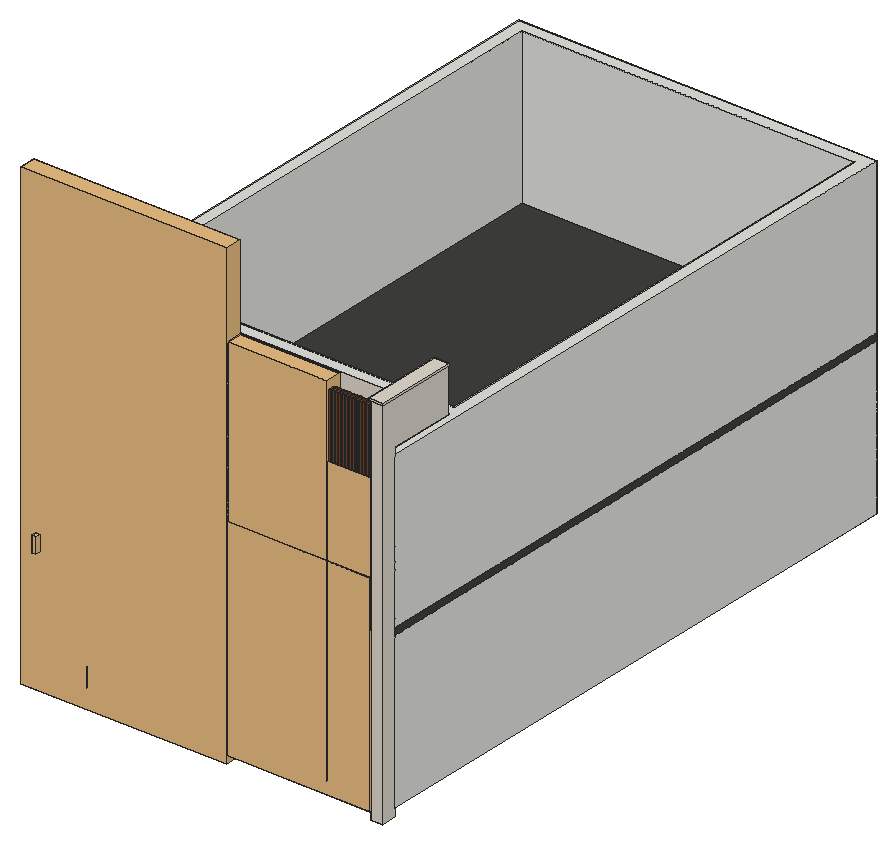
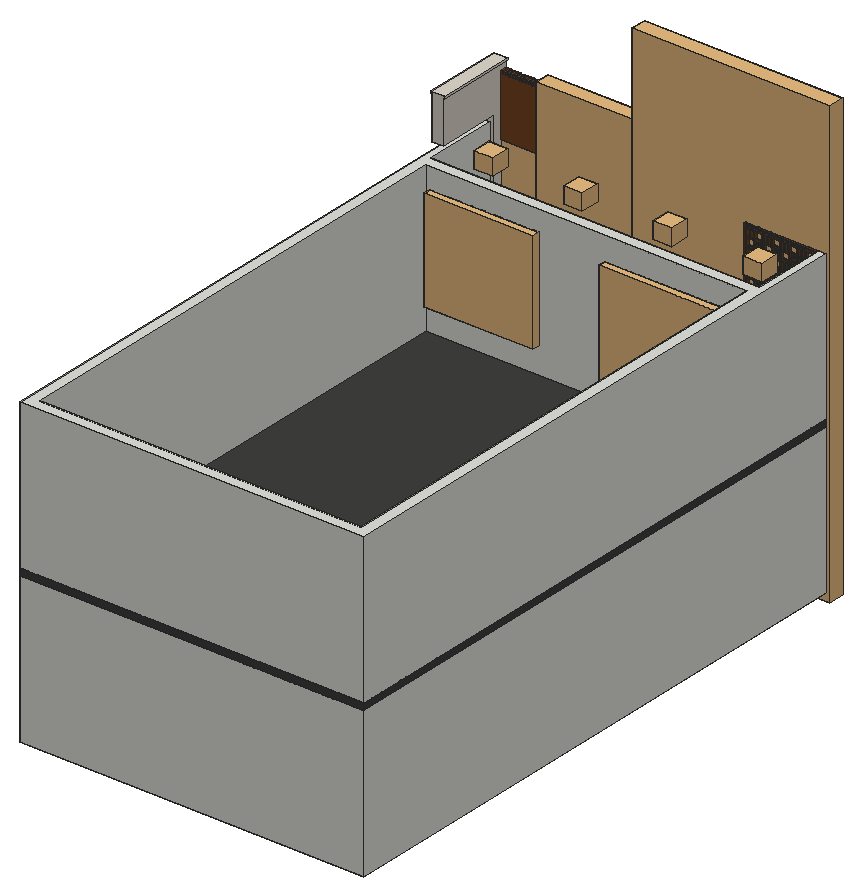
# SketchUp Ruby script. Lengths in inches.
U = 1.inch
M = Sketchup.active_model
def pt(a) = Geom::Point3d.new(a.map { |v| v * U })
def face(e, loops, mat)
  f = e.add_face(loops[0].map { |a| pt(a) })
  loops[1..].each { |l| e.add_face(l.map { |a| pt(a) }).erase! }
  f.material = f.back_material = mat if mat
  f
end
# faces: each face lists its corners as indices into pts; further lists are holes
def faces(e, pts, list, mat = nil) = list.each { |f| face(e, (f[0].is_a?(Array) ? f : [f]).map { |l| l.map { |i| pts[i] } }, mat) }
# xy, xz, yz: faces in a plane at the given z, y or x. An outline is a flat list of corners, or four numbers for a rectangle; further outlines are holes
def ring(l) = l.size == 4 ? [[l[0], l[1]], [l[2], l[1]], [l[2], l[3]], [l[0], l[3]]] : l.each_slice(2).to_a
def flat(e, list, mat, &to3) = list.each { |f| face(e, (f[0].is_a?(Array) ? f : [f]).map { |l| ring(l).map { |u, v| to3.(u, v) } }, mat) }
def xy(e, z, list, mat = nil) = flat(e, list, mat) { |x, y| [x, y, z] }
def xz(e, y, list, mat = nil) = flat(e, list, mat) { |x, z| [x, y, z] }
def yz(e, x, list, mat = nil) = flat(e, list, mat) { |y, z| [x, y, z] }
def lines(e, pts, list) = list.each { |a, b| e.add_line(pt(pts[a]), pt(pts[b])) }
# prism: a flat outline (further loops are holes) pulled along v
def prism(e, loops, v, mat = nil)
  f = face(e, loops, mat); d = Geom::Vector3d.new(v.map { |x| x * U })
  f.pushpull(f.normal.samedirection?(d) ? d.length : -d.length)
end
def box(e, o, s, mat = nil) = prism(e, [[o, [o[0] + s[0], o[1], o[2]], [o[0] + s[0], o[1] + s[1], o[2]], [o[0], o[1] + s[1], o[2]]]], [0, 0, s[2]], mat)
def at(x, y, z, deg = 0) = Geom::Transformation.translation(pt([x, y, z])) * Geom::Transformation.rotation(ORIGIN, Z_AXIS, deg.degrees)
def axes(o, x, y, z) = Geom::Transformation.new([*x, 0, *y, 0, *z, 0, *pt(o).to_a, 1])
def part(name) = M.definitions.add(name)
# library, detail: a bought-in or finely detailed component or shape, given as its bounding box
def library(name, o, s) = part(name).tap { |d| box(d.entities, o, s) }
def detail(e, o, s) = box(e.add_group.entities, o, s)
def put(e, d, t, mat = nil) = e.add_instance(d, t).tap { |i| i.material = mat if mat }
def group(e, t, mat = nil) = e.add_group.tap { |g| g.transformation = t; g.material = mat if mat }.entities
root = M.entities
M.materials.add("1448 AP 8253 RAVEN SONG").color = [64, 64, 63]
M.materials.add("[0135_DarkGray]").color = [81, 81, 81]
M.materials.add("[Concrete Stamped Ashlar]").color = [106, 67, 30]
M.materials.add("[Metal Seamed]").color = [61, 62, 60]
M.materials.add("[Steel Brushed Stainless]").color = [51, 51, 51]
M.materials.add("[Stone Vein Gray]").color = [63, 63, 63]
M.materials.add("[Tile Various Tan]").color = [223, 216, 204]
M.materials.add("[Translucent Glass Blue]1").color = [168, 168, 168]
M.materials["[Translucent Glass Blue]1"].alpha = 0.5
M.materials.add("[Translucent Glass Gray]").color = [181, 181, 181]
M.materials["[Translucent Glass Gray]"].alpha = 0.5
M.materials.add("[Translucent Glass Gray]1").color = [128, 128, 128]
M.materials["[Translucent Glass Gray]1"].alpha = 0.15
M.materials.add("[Wood Veneer 01]").color = [91, 58, 35]
M.materials.add("[Wood Veneer 01]1").color = [120, 70, 37]
c1 = library("Jaali+Partition",[0,0,0],[29.75,4.875,91.45])
c2 = library("Group\#15",[-15,-12.5,0],[147,12.5,163])
c3 = library("Group\#17",[0,0,0],[75,12,279])
c4 = library("Group\#18",[0,-3.5,0],[74,3.5,102])
c5 = library("Group\#20",[-2.91,0,-6],[155.91,13,360])
c6 = part("1")
prism(c6.entities,[[[2,-1,0],[2,1,0],[2,1,48],[2,4,48],[2,4,50],[2,-1,50]]],[-2,0,0])
c7 = library("Group\#72",[0,-2,0],[89,2,34])
c8 = part("Group\#80")
box(c8.entities,[0,-0.5,0],[24,0.5,32.25])
c9 = library("Group\#22",[0,-12.5,0],[72,12.5,15.01])
c10 = library("Curtains",[0,0,0],[121.73,8.19,117.22])
c11 = part("หน้าต่าง3บาน")
xy(c11.entities,42.78,[[77.6875,12.74,148.55,16.68]])
xy(c11.entities,43.96,[[78.87,12.74,147.37,12.74,147.37,14.71,125.72,14.71,125.72,13.13,100.52,13.13,100.52,14.71,78.87,14.71],[100.52,13.13,102.88,14.71],[123.36,13.13,125.72,14.71],[102.49,14.71,123.75,14.71,123.75,16.28,147.37,16.28,147.37,16.68,78.87,16.68,78.87,16.28,102.49,16.28]])
xy(c11.entities,45.93,[[102.49,13.13,123.75,13.92],[102.49,13.92,123.75,14.71],[80.84,14.71,100.52,15.49],[125.72,14.71,145.4,15.49],[80.84,15.49,100.52,16.28],
  [125.72,15.49,145.4,16.28]])
xy(c11.entities,83.09,[[102.49,13.13,123.75,13.92],[102.49,13.92,123.75,14.71],[80.84,14.71,100.52,15.49],[125.72,14.71,145.4,15.49],[80.84,15.49,100.52,16.28],
  [125.72,15.49,145.4,16.28]])
xy(c11.entities,84.91,[[78.87,12.74,78.87,14.71,100.52,14.71,100.52,13.13,125.72,13.13,125.72,14.71,147.37,14.71,147.37,12.74],[100.52,13.13,125.72,14.71],[102.49,14.71,102.49,16.28,78.87,16.28,78.87,16.68,147.37,16.68,147.37,16.28,123.75,16.28,123.75,14.71],[78.87,14.71,102.49,16.28]])
xy(c11.entities,86.09,[[77.6875,12.74,148.55,16.68]])
xz(c11.entities,12.74,[[[77.6875,42.78,148.55,86.09],[78.87,43.96,147.37,84.91]]])
xz(c11.entities,13.13,[[[100.52,43.96,125.72,84.91],[102.49,45.93,123.75,83.09]]])
xz(c11.entities,13.92,[[102.49,45.93,123.75,83.09]],"[Translucent Glass Blue]1")
xz(c11.entities,14.71,[[78.87,43.96,100.52,43.96,100.52,45.93,80.84,45.93,80.84,83.09,100.52,83.09,100.52,84.91,78.87,84.91],[100.52,43.96,102.49,84.91],[102.49,43.96,123.75,45.93],[125.72,43.96,147.37,43.96,147.37,84.91,125.72,84.91,125.72,83.09,145.4,83.09,145.4,45.93,125.72,45.93],[102.49,83.09,123.75,84.91]])
xz(c11.entities,15.49,[[80.44,82.9375,80.84,83.73]])
xz(c11.entities,15.49,[[80.84,45.93,100.52,83.09],[125.72,45.93,145.4,83.09]],"[Translucent Glass Blue]1")
xz(c11.entities,16.28,[[[78.87,43.96,102.49,84.91],[80.84,45.93,100.52,83.09]],[[123.75,43.96,147.37,84.91],[125.72,45.93,145.4,83.09]]])
xz(c11.entities,16.68,[[[77.6875,42.78,148.55,86.09],[78.87,43.96,147.37,84.91]]])
yz(c11.entities,77.6875,[[12.74,42.78,16.68,86.09]])
yz(c11.entities,78.87,[[12.74,43.96,14.71,84.91],[16.28,43.96,16.68,84.91]])
yz(c11.entities,80.84,[[14.71,45.93,15.49,83.09],[15.49,45.93,16.28,83.09]])
yz(c11.entities,100.52,[[13.13,43.96,14.71,84.91],[14.71,45.93,15.49,83.09],[15.49,45.93,16.28,83.09]])
yz(c11.entities,102.49,[[14.71,43.96,16.28,84.91],[13.13,45.93,13.92,83.09],[13.92,45.93,14.71,83.09]])
yz(c11.entities,123.75,[[14.71,43.96,16.28,84.91],[13.13,45.93,13.92,83.09],[13.92,45.93,14.71,83.09]])
yz(c11.entities,125.72,[[13.13,43.96,14.71,84.91],[14.71,45.93,15.49,83.09],[15.49,45.93,16.28,83.09]])
yz(c11.entities,145.4,[[14.71,45.93,15.49,83.09],[15.49,45.93,16.28,83.09]])
yz(c11.entities,147.37,[[12.74,43.96,14.71,84.91],[16.28,43.96,16.68,84.91]])
yz(c11.entities,148.55,[[12.74,42.78,16.68,86.09]])
p = [[80.44,15.49,84.91],[80.44,15.49,83.73]]
lines(c11.entities,p,[[0,1]])
c12 = library("AS-120-mm\#1",[0,0,0],[49.44,4.72,60])
c13 = library("WALL LIGHT 69",[4.19,4.05,-8.78],[4.61,5.7,17.13])
c14 = part("Group\#81")
prism(c14.entities,[[[8,8,0],[8,0,0],[0,0,0],[0,8,0]],[[4.25,3.75,0],[4.25,0.5,0],[7.5,0.5,0],[7.5,3.75,0]],[[0.5,7.5,0],[0.5,4.25,0],[3.75,4.25,0],[3.75,7.5,0]],[[5.625,4.25,0],[5.625,7.5,0],[4.25,7.5,0],[4.25,4.25,0]],[[7.5,7.5,0],[6.125,7.5,0],[6.125,4.25,0],[7.5,4.25,0]],[[0.5,3.75,0],[0.5,2.375,0],[3.75,2.375,0],[3.75,3.75,0]],[[0.5,0.5,0],[3.75,0.5,0],[3.75,1.875,0],[0.5,1.875,0]]],[0,0,3])
c15 = part("contemporary square jaali - swamy and co")
g1 = group(c15.entities,at(69.36,8.01,-1.33))
put(g1,c14,axes([24,1.28,40],[1,0,0],[0,0,1],[0,-0.42667,0]),"[Concrete Stamped Ashlar]")
put(g1,c14,axes([0,1.28,48],[1,0,0],[0,0,1],[0,-0.42667,0]),"[Concrete Stamped Ashlar]")
put(g1,c14,axes([8,1.28,40],[1,0,0],[0,0,1],[0,-0.42667,0]),"[Concrete Stamped Ashlar]")
put(g1,c14,axes([16,1.28,40],[1,0,0],[0,0,1],[0,-0.42667,0]),"[Concrete Stamped Ashlar]")
put(g1,c14,axes([8,1.28,48],[1,0,0],[0,0,1],[0,-0.42667,0]),"[Concrete Stamped Ashlar]")
put(g1,c14,axes([24,1.28,48],[1,0,0],[0,0,1],[0,-0.42667,0]),"[Concrete Stamped Ashlar]")
put(g1,c14,axes([16,1.28,48],[1,0,0],[0,0,1],[0,-0.42667,0]),"[Concrete Stamped Ashlar]")
put(g1,c14,axes([0,1.28,32],[1,0,0],[0,0,1],[0,-0.42667,0]),"[Concrete Stamped Ashlar]")
put(g1,c14,axes([8,1.28,24],[1,0,0],[0,0,1],[0,-0.42667,0]),"[Concrete Stamped Ashlar]")
put(g1,c14,axes([16,1.28,24],[1,0,0],[0,0,1],[0,-0.42667,0]),"[Concrete Stamped Ashlar]")
put(g1,c14,axes([24,1.28,24],[1,0,0],[0,0,1],[0,-0.42667,0]),"[Concrete Stamped Ashlar]")
put(g1,c14,axes([24,1.28,56],[1,0,0],[0,0,1],[0,-0.42667,0]),"[Concrete Stamped Ashlar]")
put(g1,c14,axes([16,1.28,8],[1,0,0],[0,0,1],[0,-0.42667,0]),"[Concrete Stamped Ashlar]")
put(g1,c14,axes([0,1.28,24],[1,0,0],[0,0,1],[0,-0.42667,0]),"[Concrete Stamped Ashlar]")
put(g1,c14,axes([0,1.28,16],[1,0,0],[0,0,1],[0,-0.42667,0]),"[Concrete Stamped Ashlar]")
put(g1,c14,axes([24,1.28,8],[1,0,0],[0,0,1],[0,-0.42667,0]),"[Concrete Stamped Ashlar]")
put(g1,c14,axes([8,1.28,16],[1,0,0],[0,0,1],[0,-0.42667,0]),"[Concrete Stamped Ashlar]")
put(g1,c14,axes([16,1.28,16],[1,0,0],[0,0,1],[0,-0.42667,0]),"[Concrete Stamped Ashlar]")
put(g1,c14,axes([24,1.28,16],[1,0,0],[0,0,1],[0,-0.42667,0]),"[Concrete Stamped Ashlar]")
put(g1,c14,axes([0,1.28,56],[1,0,0],[0,0,1],[0,-0.42667,0]),"[Concrete Stamped Ashlar]")
put(g1,c14,axes([24,1.28,32],[1,0,0],[0,0,1],[0,-0.42667,0]),"[Concrete Stamped Ashlar]")
put(g1,c14,axes([16,1.28,32],[1,0,0],[0,0,1],[0,-0.42667,0]),"[Concrete Stamped Ashlar]")
put(g1,c14,axes([0,1.28,40],[1,0,0],[0,0,1],[0,-0.42667,0]),"[Concrete Stamped Ashlar]")
put(g1,c14,axes([8,1.28,32],[1,0,0],[0,0,1],[0,-0.42667,0]),"[Concrete Stamped Ashlar]")
put(g1,c14,axes([0,1.28,0],[1,0,0],[0,0,1],[0,-0.42667,0]),"[Concrete Stamped Ashlar]")
put(g1,c14,axes([0,1.28,8],[1,0,0],[0,0,1],[0,-0.42667,0]),"[Concrete Stamped Ashlar]")
put(g1,c14,axes([16,1.28,56],[1,0,0],[0,0,1],[0,-0.42667,0]),"[Concrete Stamped Ashlar]")
put(g1,c14,axes([8,1.28,0],[1,0,0],[0,0,1],[0,-0.42667,0]),"[Concrete Stamped Ashlar]")
put(g1,c14,axes([16,1.28,0],[1,0,0],[0,0,1],[0,-0.42667,0]),"[Concrete Stamped Ashlar]")
put(g1,c14,axes([24,1.28,0],[1,0,0],[0,0,1],[0,-0.42667,0]),"[Concrete Stamped Ashlar]")
put(g1,c14,axes([8,1.28,56],[1,0,0],[0,0,1],[0,-0.42667,0]),"[Concrete Stamped Ashlar]")
put(g1,c14,axes([8,1.28,8],[1,0,0],[0,0,1],[0,-0.42667,0]),"[Concrete Stamped Ashlar]")
g2 = group(c15.entities,at(67.86,7.61,-2.83),"[Wood Veneer 01]")
xy(g2,0.5,[[0.5,0,34.5,2]])
xy(g2,1.5,[[1.5,0,33.5,2]])
xy(g2,65.5,[[1.5,0,33.5,2]])
xy(g2,66.5,[[0.5,0,34.5,2]])
xz(g2,0,[[[0.5,0.5,34.5,66.5],[1.5,1.5,33.5,65.5]]])
yz(g2,0.5,[[0,0.5,2,66.5]])
yz(g2,1.5,[[0,1.5,2,65.5]])
yz(g2,33.5,[[0,1.5,2,65.5]])
yz(g2,34.5,[[0,0.5,2,66.5]])
c16 = part("PENTEK_RP Fineline 50S_Sliding_DoorCase_E1")
box(c16.entities,[0,0,0],[1.51,3.66,99.27],"[0135_DarkGray]")
c17 = part("PENTEK_RP Fineline 50S_SlidingDooe_Case_E2")
box(c17.entities,[0,0,0],[96.25,3.66,1.51],"[0135_DarkGray]")
c18 = part("pentek_RP Fineline 50S_SlidingDoor_Case")
put(c18.entities,c16,at(97.76,0,0))
put(c18.entities,c17,at(1.51,0,0))
put(c18.entities,c16,at(0,0,0))
put(c18.entities,c17,at(1.51,0,97.76))
c19 = part("PENTEK_RP Fineline 50S_SlidingDoor_GlazingBead_2")
box(c19.entities,[0,0,0],[0.56,0.59,94.39],"[0135_DarkGray]")
c20 = part("PENTEK_RP Fineline 50S_SlidingDoor_Glass")
box(c20.entities,[0,0,0],[46.58,0.16,94.39],"[Translucent Glass Gray]1")
c21 = part("PENTEK_RP Fineline 50S_SlidingDoor_GlazingBead")
box(c21.entities,[0,0,0],[45.47,0.59,0.56],"[0135_DarkGray]")
c22 = part("PENTEK_RP Fineline 50S_SlidingDoor_Leaf_E1")
xy(c22.entities,0,[[0,0,0.93,1.97],[0.93,1.57,1.49,1.97]],"[0135_DarkGray]")
xy(c22.entities,96.25,[[0,0,0.93,0,0.93,1.57,1.49,1.57,1.49,1.97,0,1.97]],"[0135_DarkGray]")
xz(c22.entities,0,[[0,0,0.93,96.25]],"[0135_DarkGray]")
xz(c22.entities,1.57,[[0.93,0,1.49,95.32],[0.93,95.32,1.49,96.25]],"[0135_DarkGray]")
xz(c22.entities,1.97,[[0,0,1.49,96.25]],"[0135_DarkGray]")
yz(c22.entities,0,[[0,0,1.97,96.25]],"[0135_DarkGray]")
yz(c22.entities,0.93,[[0,0,1.57,0.93],[0,0.93,1.57,95.32],[0,95.32,1.57,96.25]],"[0135_DarkGray]")
yz(c22.entities,1.49,[[1.57,0,1.97,95.32],[1.57,95.32,1.97,96.25]],"[0135_DarkGray]")
c23 = part("PENTEK_RP Fineline 50S_SlidingDoor_Leaf_E2")
xy(c23.entities,0,[[0,0,0,1.57,0.56,1.57,0.56,1.97,46.02,1.97,46.02,1.57,46.58,1.57,46.58,0]],"[0135_DarkGray]")
xy(c23.entities,0.93,[[0,0,46.58,1.57]],"[0135_DarkGray]")
xy(c23.entities,1.49,[[0.56,1.57,46.02,1.97]],"[0135_DarkGray]")
xz(c23.entities,0,[[0,0,46.58,0.93]],"[0135_DarkGray]")
xz(c23.entities,1.57,[[0,0,0.56,0.93],[46.02,0,46.58,0.93],[0.56,0.93,46.02,1.49]],"[0135_DarkGray]")
xz(c23.entities,1.97,[[0.56,0,46.02,1.49]],"[0135_DarkGray]")
yz(c23.entities,0,[[0,0,1.57,0.93]],"[0135_DarkGray]")
yz(c23.entities,0.56,[[1.57,0,1.97,0.93],[1.57,0.93,1.97,1.49]],"[0135_DarkGray]")
yz(c23.entities,46.02,[[1.57,0,1.97,0.93],[1.57,0.93,1.97,1.49]],"[0135_DarkGray]")
yz(c23.entities,46.58,[[0,0,1.57,0.93]],"[0135_DarkGray]")
c24 = part("PENTEK_RP Fineline S_SlidingDoor_Leaf1")
put(c24.entities,c19,at(0.93,0,0.93))
put(c24.entities,c19,at(46.96,0,0.93))
put(c24.entities,c20,at(1.49,1.42,0.93))
put(c24.entities,c21,at(1.49,0,0.93))
put(c24.entities,c20,at(1.49,0.59,0.93))
put(c24.entities,c22,at(0,0,0))
put(c24.entities,c22,axes([48.44,0,0],[-1,0,0],[0,1,0],[0,0,1]))
put(c24.entities,c23,axes([0.93,0,96.25],[1,0,0],[0,1,0],[0,0,-1]))
put(c24.entities,c23,at(0.93,0,0))
put(c24.entities,c21,at(1.49,0,94.77))
c25 = part("PENTEK_RP Fineline 50S_SlidingDoor_Leaf2")
put(c25.entities,c20,at(1.49,1.42,0.93))
put(c25.entities,c21,at(1.49,0,94.77))
put(c25.entities,c19,at(46.96,0,0.93))
put(c25.entities,c20,at(1.49,0.59,0.93))
put(c25.entities,c19,at(0.93,0,0.93))
put(c25.entities,c22,at(0,0,0))
put(c25.entities,c22,axes([48.44,0,0],[-1,0,0],[0,1,0],[0,0,1]))
put(c25.entities,c21,at(1.49,0,0.93))
put(c25.entities,c23,axes([0.93,0,96.25],[1,0,0],[0,1,0],[0,0,-1]))
put(c25.entities,c23,at(0.93,0,0))
c26 = part("PENTEK_RP+Fineline+50S_Sliding_Door (1)")
put(c26.entities,c18,at(0,-1.88,-0.09))
put(c26.entities,c24,at(1.51,-2.27,1.42))
put(c26.entities,c25,at(49.32,-0.3,1.42))
c27 = library("AS-120-mm",[0,0,0],[49.44,4.72,66.14])
c28 = library("11",[-5.64,-5.64,-13.23],[15.28,15.28,13.23])
xy(root,123,[[39.35,204,39.27,204.01,39.19,204.01,39.12,204.02,38.88,204.05,38.81,204.07,38.65,204.11,38.58,204.13,38.5,204.15,38.36,204.21,38.28,204.24,38.14,204.3,38.07,204.34,37.93,204.41,37.87,204.45,37.8,204.5,37.73,204.54,37.67,204.59,37.61,204.63,37.43,204.78,37.37,204.84,37.3125,204.89,37.26,204.95,37.01,205.25,36.97,205.32,36.92,205.38,36.8,205.59,36.77,205.66,36.73,205.73,36.64,205.94,36.62,206.02,36.59,206.09,36.57,206.17,36.55,206.24,36.51,206.4,36.5,206.47,36.48,206.55,36.46,206.71,36.46,206.79,36.45,206.86,36.45,207.1,36.46,207.18,36.46,207.26,36.47,207.33,36.5,207.57,36.52,207.64,36.56,207.8,36.58,207.87,36.6,207.95,36.66,208.09,36.6875,208.17,36.72,208.24,36.75,208.31,36.79,208.38,36.82,208.45,36.86,208.52,36.9,208.58,36.95,208.65,36.99,208.72,37.04,208.78,37.08,208.84,37.23,209.02,37.29,209.08,37.34,209.14,37.64,209.39,37.7,209.4375,37.77,209.48,37.83,209.53,38.04,209.65,38.11,209.68,38.18,209.72,38.39,209.81,38.47,209.83,38.54,209.86,38.62,209.88,38.69,209.9,38.77,209.92,38.85,209.9375,38.92,209.95,39,209.97,39.16,209.99,39.24,209.99,39.3125,210,39.55,210,39.63,209.99,39.71,209.99,39.78,209.98,40.02,209.95,40.09,209.93,40.25,209.89,40.32,209.87,40.4,209.85,40.54,209.79,40.62,209.76,40.6875,209.73,40.76,209.7,40.83,209.66,40.97,209.59,41.03,209.55,41.1,209.5,41.17,209.46,41.23,209.41,41.29,209.37,41.47,209.22,41.53,209.16,41.59,209.11,41.89,208.75,41.93,208.68,41.98,208.62,42.1,208.41,42.13,208.34,42.17,208.27,42.26,208.06,42.28,207.98,42.31,207.91,42.33,207.83,42.35,207.76,42.39,207.6,42.4,207.53,42.42,207.45,42.43,207.37,42.4375,207.29,42.44,207.21,42.45,207.14,42.45,206.9,42.44,206.82,42.4375,206.74,42.43,206.67,42.4,206.43,42.38,206.36,42.34,206.2,42.32,206.13,42.3,206.05,42.24,205.91,42.21,205.83,42.15,205.69,42.11,205.62,42.08,205.55,42.04,205.48,42,205.42,41.95,205.35,41.91,205.28,41.86,205.22,41.82,205.16,41.67,204.98,41.61,204.92,41.56,204.86,41.26,204.61,41.2,204.5625,41.13,204.52,41.07,204.47,40.86,204.35,40.79,204.32,40.72,204.28,40.51,204.19,40.43,204.17,40.36,204.14,40.28,204.12,40.21,204.1,40.13,204.08,40.05,204.0625,39.98,204.05,39.9,204.03,39.74,204.01,39.66,204.01,39.59,204],[77.87,204,77.79,204.01,77.71,204.01,77.64,204.02,77.4,204.05,77.33,204.07,77.17,204.11,77.1,204.13,77.02,204.15,76.95,204.18,76.8,204.24,76.66,204.3,76.59,204.34,76.45,204.41,76.39,204.45,76.32,204.5,76.25,204.54,76.19,204.59,76.13,204.63,75.95,204.78,75.89,204.84,75.83,204.89,75.68,205.07,75.625,205.13,75.58,205.19,75.53,205.25,75.49,205.32,75.44,205.38,75.32,205.59,75.29,205.66,75.25,205.73,75.16,205.94,75.14,206.02,75.11,206.09,75.09,206.17,75.07,206.24,75.03,206.4,75.02,206.47,75,206.55,74.98,206.71,74.98,206.79,74.97,206.86,74.97,207.1,74.98,207.18,74.98,207.26,74.99,207.33,75.02,207.57,75.04,207.64,75.08,207.8,75.1,207.87,75.125,207.95,75.15,208.02,75.18,208.09,75.21,208.17,75.27,208.31,75.31,208.38,75.34,208.45,75.38,208.52,75.42,208.58,75.47,208.65,75.51,208.72,75.56,208.78,75.6,208.84,75.75,209.02,75.81,209.08,75.86,209.14,76.16,209.39,76.22,209.4375,76.29,209.48,76.35,209.53,76.56,209.65,76.625,209.68,76.7,209.72,76.91,209.81,76.99,209.83,77.0625,209.86,77.14,209.88,77.21,209.9,77.29,209.92,77.37,209.9375,77.44,209.95,77.52,209.97,77.68,209.99,77.76,209.99,77.83,210,78.07,210,78.15,209.99,78.23,209.99,78.3,209.98,78.54,209.95,78.61,209.93,78.77,209.89,78.84,209.87,78.92,209.85,78.99,209.82,79.0625,209.79,79.14,209.76,79.28,209.7,79.35,209.66,79.49,209.59,79.55,209.55,79.62,209.5,79.6875,209.46,79.75,209.41,79.8125,209.37,79.875,209.32,79.93,209.27,79.99,209.22,80.05,209.16,80.11,209.11,80.26,208.93,80.3125,208.87,80.36,208.81,80.41,208.75,80.45,208.68,80.5,208.62,80.62,208.41,80.65,208.34,80.6875,208.27,80.72,208.2,80.78,208.06,80.8,207.98,80.83,207.91,80.85,207.83,80.875,207.76,80.89,207.68,80.91,207.6,80.92,207.53,80.9375,207.45,80.95,207.37,80.96,207.29,80.96,207.21,80.97,207.14,80.97,206.9,80.96,206.82,80.96,206.74,80.95,206.67,80.92,206.43,80.9,206.36,80.86,206.2,80.84,206.13,80.82,206.05,80.76,205.91,80.73,205.83,80.67,205.69,80.63,205.62,80.6,205.55,80.56,205.48,80.52,205.42,80.47,205.35,80.43,205.28,80.38,205.22,80.34,205.16,80.24,205.04,80.1875,204.98,80.13,204.92,80.08,204.86,79.78,204.61,79.72,204.5625,79.65,204.52,79.59,204.47,79.38,204.35,79.3125,204.32,79.24,204.28,79.03,204.19,78.95,204.17,78.88,204.14,78.8,204.12,78.73,204.1,78.65,204.08,78.57,204.0625,78.5,204.05,78.42,204.03,78.26,204.01,78.18,204.01,78.11,204]],"1448 AP 8253 RAVEN SONG")
xy(root,126,[[9.27,183,278.1,183,278.1,195,287.37,195,287.37,663,9.27,663]],"1448 AP 8253 RAVEN SONG")
xz(root,209.99,[[39.16,120,39.24,123],[39.63,120,39.71,123]],"1448 AP 8253 RAVEN SONG")
xz(root,210,[[39.3125,120,39.39,123],[39.39,120,39.47,123],[39.47,120,39.55,123]],"1448 AP 8253 RAVEN SONG")
yz(root,36.45,[[206.86,120,206.94,123],[206.94,120,207.02,123],[207.02,120,207.1,123]],"1448 AP 8253 RAVEN SONG")
yz(root,36.46,[[206.71,120,206.79,123],[207.18,120,207.26,123]],"1448 AP 8253 RAVEN SONG")
p = [[37.06,205.19,120],[37.01,205.25,120],[37.01,205.25,123],[37.06,205.19,123],[36.97,205.32,120],[36.92,205.38,120],
  [36.92,205.38,123],[36.97,205.32,123],[36.88,205.45,120],[36.88,205.45,123],[36.84,205.52,120],[36.84,205.52,123],
  [36.8,205.59,120],[36.8,205.59,123],[36.77,205.66,120],[36.77,205.66,123],[36.73,205.73,120],[36.73,205.73,123],
  [36.7,205.8,120],[36.7,205.8,123],[36.67,205.87,120],[36.67,205.87,123],[36.64,205.94,120],[36.64,205.94,123],
  [36.62,206.02,120],[36.62,206.02,123],[36.59,206.09,120],[36.59,206.09,123],[36.57,206.17,120],[36.57,206.17,123],
  [36.55,206.24,120],[36.55,206.24,123],[36.53,206.32,120],[36.53,206.32,123],[36.51,206.4,120],[36.51,206.4,123],
  [36.5,206.47,120],[36.5,206.47,123],[36.48,206.55,120],[36.48,206.55,123],[36.47,206.63,120],[36.47,206.63,123],
  [36.46,206.71,120],[36.46,206.71,123],[36.46,206.79,120],[36.45,206.86,120],[36.45,206.86,123],[36.46,206.79,123],
  [36.45,207.1,120],[36.46,207.18,120],[36.46,207.18,123],[36.45,207.1,123],[36.46,207.26,120],[36.47,207.33,120],
  [36.47,207.33,123],[36.46,207.26,123],[36.48,207.41,120],[36.48,207.41,123],[36.49,207.49,120],[36.49,207.49,123],
  [36.5,207.57,120],[36.5,207.57,123],[36.52,207.64,120],[36.52,207.64,123],[36.54,207.72,120],[36.54,207.72,123],
  [36.56,207.8,120],[36.56,207.8,123],[36.58,207.87,120],[36.58,207.87,123],[36.6,207.95,120],[36.6,207.95,123],
  [36.63,208.02,120],[36.63,208.02,123],[36.66,208.09,120],[36.66,208.09,123],[36.6875,208.17,120],[36.6875,208.17,123],
  [36.72,208.24,120],[36.72,208.24,123],[36.75,208.31,120],[36.75,208.31,123],[36.79,208.38,120],[36.79,208.38,123],
  [36.82,208.45,120],[36.82,208.45,123],[36.86,208.52,120],[36.86,208.52,123],[36.9,208.58,120],[36.9,208.58,123],
  [36.95,208.65,120],[36.95,208.65,123],[36.99,208.72,120],[36.99,208.72,123],[37.04,208.78,120],[37.04,208.78,123],
  [37.08,208.84,120],[37.08,208.84,123],[37.13,208.9,120],[37.13,208.9,123],[37.18,208.96,120],[37.18,208.96,123],
  [37.23,209.02,120],[37.23,209.02,123],[37.29,209.08,120],[37.29,209.08,123],[37.34,209.14,120],[37.34,209.14,123],
  [37.4,209.19,120],[37.4,209.19,123],[37.46,209.24,120],[37.46,209.24,123],[37.52,209.29,120],[37.52,209.29,123],
  [37.58,209.34,120],[37.58,209.34,123],[37.64,209.39,120],[37.64,209.39,123],[37.7,209.4375,120],[37.7,209.4375,123],
  [37.77,209.48,120],[37.77,209.48,123],[41.17,209.46,120],[41.23,209.41,120],[41.23,209.41,123],[41.17,209.46,123],
  [37.83,209.53,120],[37.83,209.53,123],[37.9,209.57,120],[37.9,209.57,123],[40.97,209.59,120],[41.03,209.55,120],
  [41.03,209.55,123],[40.97,209.59,123],[41.1,209.5,120],[41.1,209.5,123],[37.97,209.61,120],[37.97,209.61,123],
  [38.04,209.65,120],[38.04,209.65,123],[38.11,209.68,120],[38.11,209.68,123],[40.83,209.66,120],[40.9,209.625,120],
  [40.9,209.625,123],[40.83,209.66,123],[38.18,209.72,120],[38.18,209.72,123],[38.25,209.75,120],[38.25,209.75,123],
  [38.32,209.78,120],[38.32,209.78,123],[40.62,209.76,120],[40.6875,209.73,120],[40.6875,209.73,123],[40.62,209.76,123],
  [40.76,209.7,120],[40.76,209.7,123],[38.39,209.81,120],[38.39,209.81,123],[38.47,209.83,120],[38.47,209.83,123],
  [38.54,209.86,120],[38.54,209.86,123],[40.32,209.87,120],[40.4,209.85,120],[40.4,209.85,123],[40.32,209.87,123],
  [40.47,209.82,120],[40.47,209.82,123],[40.54,209.79,120],[40.54,209.79,123],[38.62,209.88,120],[38.62,209.88,123],
  [38.69,209.9,120],[38.69,209.9,123],[38.77,209.92,120],[38.77,209.92,123],[38.85,209.9375,120],[38.85,209.9375,123],
  [38.92,209.95,120],[38.92,209.95,123],[39.94,209.96,120],[40.02,209.95,120],[40.02,209.95,123],[39.94,209.96,123],
  [40.09,209.93,120],[40.09,209.93,123],[40.17,209.91,120],[40.17,209.91,123],[40.25,209.89,120],[40.25,209.89,123],
  [39,209.97,120],[39,209.97,123],[39.08,209.98,120],[39.08,209.98,123],[39.16,209.99,120],[39.16,209.99,123],
  [39.24,209.99,120],[39.3125,210,120],[39.3125,210,123],[39.24,209.99,123],[39.55,210,120],[39.63,209.99,120],
  [39.63,209.99,123],[39.55,210,123],[39.71,209.99,120],[39.78,209.98,120],[39.78,209.98,123],[39.71,209.99,123],
  [39.86,209.97,120],[39.86,209.97,123]]
faces(root,p,[[0,1,2,3],[4,5,6,7],[1,4,7,2],[5,8,9,6],[8,10,11,9],[10,12,13,11],[12,14,15,13],[14,16,17,15],
  [16,18,19,17],[18,20,21,19],[20,22,23,21],[22,24,25,23],[24,26,27,25],[26,28,29,27],[28,30,31,29],[30,32,33,31],
  [32,34,35,33],[34,36,37,35],[36,38,39,37],[38,40,41,39],[40,42,43,41],[44,45,46,47],[48,49,50,51],[52,53,54,55],
  [53,56,57,54],[56,58,59,57],[58,60,61,59],[60,62,63,61],[62,64,65,63],[64,66,67,65],[66,68,69,67],[68,70,71,69],
  [70,72,73,71],[72,74,75,73],[74,76,77,75],[76,78,79,77],[78,80,81,79],[80,82,83,81],[82,84,85,83],[84,86,87,85],
  [86,88,89,87],[88,90,91,89],[90,92,93,91],[92,94,95,93],[94,96,97,95],[96,98,99,97],[98,100,101,99],[100,102,103,101],
  [102,104,105,103],[104,106,107,105],[106,108,109,107],[108,110,111,109],[110,112,113,111],[112,114,115,113],[114,116,117,115],[116,118,119,117],
  [118,120,121,119],[122,123,124,125],[120,126,127,121],[126,128,129,127],[130,131,132,133],[131,134,135,132],[134,122,125,135],[128,136,137,129],
  [136,138,139,137],[138,140,141,139],[142,143,144,145],[143,130,133,144],[140,146,147,141],[146,148,149,147],[148,150,151,149],[152,153,154,155],
  [153,156,157,154],[156,142,145,157],[150,158,159,151],[158,160,161,159],[160,162,163,161],[164,165,166,167],[165,168,169,166],[168,170,171,169],
  [170,152,155,171],[162,172,173,163],[172,174,175,173],[174,176,177,175],[176,178,179,177],[178,180,181,179],[182,183,184,185],[183,186,187,184],
  [186,188,189,187],[188,190,191,189],[190,164,167,191],[180,192,193,181],[192,194,195,193],[194,196,197,195],[198,199,200,201],[202,203,204,205],
  [206,207,208,209],[207,210,211,208],[210,182,185,211]],"1448 AP 8253 RAVEN SONG")
g3 = group(root,at(9.27,183,126))
xy(g3,0,[[[0,12,278.1,480],[9.27,21,268.83,471]]])
xy(g3,30,[[49.44,12,123.6,21],[176.13,12,225.57,21]])
xy(g3,90,[[49.44,12,123.6,21],[176.13,12,225.57,21]])
xy(g3,120,[[[0,12,278.1,480],[9.27,21,268.83,471]]])
xz(g3,12,[[[0,0,278.1,120],[49.44,30,123.6,90],[176.13,30,225.57,90]]],"[Tile Various Tan]")
xz(g3,21,[[[9.27,0,268.83,120],[49.44,30,123.6,90],[176.13,30,225.57,90]]])
xz(g3,471,[[9.27,0,268.83,120]])
xz(g3,480,[[0,0,278.1,120]])
yz(g3,0,[[12,0,480,120]])
yz(g3,9.27,[[21,0,471,120]])
yz(g3,49.44,[[12,30,21,90]])
yz(g3,123.6,[[12,30,21,90]])
yz(g3,176.13,[[12,30,21,90]])
yz(g3,225.57,[[12,30,21,90]])
yz(g3,268.83,[[21,0,471,120]])
yz(g3,278.1,[[12,0,480,120]])
g4 = group(g3,at(0,12,0),"[Tile Various Tan]")
xy(g4,-6,[[268.83,-12,278.1,0]])
xy(g4,252,[[268.83,0,278.1,51]])
xy(g4,286.5,[[267.8,-13,267.8,51,268.83,51,268.83,-12,278.1,-12,278.1,51,279.13,51,279.13,-13]])
xy(g4,288,[[267.8,-13,279.13,51]])
xz(g4,-13,[[267.8,286.5,279.13,288]])
xz(g4,-12,[[268.83,-6,278.1,286.5]],"[Tile Various Tan]")
xz(g4,0,[[268.83,-6,278.1,252]])
xz(g4,51,[[268.83,252,278.1,288],[267.8,286.5,268.83,288],[278.1,286.5,279.13,288]])
yz(g4,267.8,[[-13,286.5,51,288]])
yz(g4,268.83,[[-12,-6,-12,286.5,51,286.5,51,252,0,252,0,-6]],"[Tile Various Tan]")
yz(g4,278.1,[[-12,-6,0,-6,0,252,51,252,51,286.5,-12,286.5]])
yz(g4,279.13,[[-13,286.5,51,288]])
p = [[123.6,0,90],[123.6,0,30],[176.13,0,30],[176.13,0,90],[225.57,0,90],[225.57,0,30]]
lines(g4,p,[[0,1],[2,3],[4,3],[5,4],[2,5]])
put(g4,c1,axes([234.84,-12,126],[1.14262,0,0],[0,1,0],[0,0,1.15906]))
put(g4,c2,axes([132.87,0,0],[1.03,0,0],[0,1,0],[0,0,1]),"[Stone Vein Gray]")
put(g4,c3,axes([157.59,-12,9],[1.03,0,0],[0,1,0],[0,0,1]))
put(g4,c4,axes([176.13,0,9],[1.03,0,0],[0,1,0],[0,0,1]),"[Wood Veneer 01]1")
g5 = group(g4,at(176.13,0,9),"[Tile Various Tan]")
detail(g5,[0,-10.5,0],[92.7,10.5,117])
put(g4,c5,axes([0,-13,0],[1.03,0,0],[0,1,0],[0,0,1]))
g6 = group(g4,at(132.87,-13,0),"[Tile Various Tan]")
box(g6,[-108.15,1,0],[108.15,11,8.99])
g7 = group(g4,at(234.84,-12,232),"[Wood Veneer 01]1")
xy(g7,0,[[0,3,33.99,6]])
xy(g7,48,[[0,3,33.99,6]])
xz(g7,3,[[0,0,33.99,48]])
xz(g7,6,[[0,0,33.99,48]])
yz(g7,0,[[3,0,6,48]])
yz(g7,33.99,[[3,0,6,48]])
put(g7,c6,axes([0,2,0],[1.11023,0,0],[0,1,0],[0,0,1]))
put(g7,c6,axes([2.65,2,0],[1.11023,0,0],[0,1,0],[0,0,1]))
put(g7,c6,axes([5.29,2,0],[1.11023,0,0],[0,1,0],[0,0,1]))
put(g7,c6,axes([7.94,2,0],[1.11023,0,0],[0,1,0],[0,0,1]))
put(g7,c6,axes([10.59,2,0],[1.11023,0,0],[0,1,0],[0,0,1]))
put(g7,c6,axes([13.24,2,0],[1.11023,0,0],[0,1,0],[0,0,1]))
put(g7,c6,axes([15.88,2,0],[1.11023,0,0],[0,1,0],[0,0,1]))
put(g7,c6,axes([18.53,2,0],[1.11023,0,0],[0,1,0],[0,0,1]))
put(g7,c6,axes([21.18,2,0],[1.11023,0,0],[0,1,0],[0,0,1]))
put(g7,c6,axes([23.83,2,0],[1.11023,0,0],[0,1,0],[0,0,1]))
put(g7,c6,axes([26.47,2,0],[1.11023,0,0],[0,1,0],[0,0,1]))
put(g7,c6,axes([29.12,2,0],[1.11023,0,0],[0,1,0],[0,0,1]))
put(g7,c6,axes([31.77,2,0],[1.11023,0,0],[0,1,0],[0,0,1]))
put(g4,c7,axes([25.75,-6,126],[1.03,0,0],[0,1,0],[0,0,1]))
g8 = group(g4,at(25.75,-9,252))
g9 = group(g8,at(0,0.5,32),"[Steel Brushed Stainless]")
prism(g9,[[[0,0,2],[0,0,0],[0,-0.75,0],[0,-0.75,0.25],[0,-1.25,0.25],[0,-1.25,0],[0,-2,0],[0,-2,2]]],[88.58,0,0])
g10 = group(g8,at(0,-0.25,0),"[Translucent Glass Gray]")
xy(g10,0,[[0,-0.47,88.58,0]])
xy(g10,32.25,[[0,-0.47,88.58,0]])
xz(g10,-0.47,[[0,0,88.58,32.25]])
xz(g10,0,[[0,0,88.58,32.25]])
yz(g10,0,[[-0.47,0,0,32.25]])
yz(g10,88.58,[[-0.47,0,0,32.25]])
g11 = group(g8,at(110.12,-2,0))
g12 = group(g11,at(0,2,32),"[Steel Brushed Stainless]")
prism(g12,[[[0,0,2],[0,0,0],[0,-0.75,0],[0,-0.75,0.25],[0,-1.25,0.25],[0,-1.25,0],[0,-2,0],[0,-2,2]]],[21.72,0,0])
put(g11,c8,axes([0,1.25,0],[0.905,0,0],[0,1,0],[0,0,1]),"[Translucent Glass Gray]")
put(g4,c8,axes([177.6875,-7.55,126],[1.93069,0,0],[0,1,0],[0,0,1]),"[Translucent Glass Gray]")
g13 = group(g4,at(177.6875,-6.8,158),"[Steel Brushed Stainless]")
prism(g13,[[[0,0,2],[0,0,0],[0,-0.75,0],[0,-0.75,0.25],[0,-1.25,0.25],[0,-1.25,0],[0,-2,0],[0,-2,2]]],[46.34,0,0])
put(g3,c9,axes([48.7,12,8.99],[1.06111,0,0],[0,1,0],[0,0,1.02]),"[Wood Veneer 01]1")
put(root,c10,axes([166.88,204,139.96],[0.721,0,0],[0,0.7,0],[0,0,0.7]))
put(root,c10,axes([52.66,204,140.04],[0.721,0,0],[0,0.7,0],[0,0,0.7]))
put(root,c11,axes([-22.59,178.49,96.73],[1.04648,0,0],[0,1.35,0],[0,0,1.38545]),"[Metal Seamed]")
put(root,c12,at(185.4,197,156),"[Metal Seamed]")
put(root,c13,axes([243.87,184.68,184.42],[0.7,0,0],[0,0.7,0],[0,0,0.7]))
put(root,c13,axes([15.53,175.18,223.42],[0.7,0,0],[0,0.7,0],[0,0,0.7]))
g14 = group(root,at(9.27,195,246),"1448 AP 8253 RAVEN SONG")
box(g14,[0,0,0],[278.1,468,6])
put(root,c15,axes([-103.2,187.39,256.23],[1.73559,0,0],[0,1,0],[0,0,1.81818]))
put(root,c10,axes([28.98,264,252],[0.85655,0,0],[0,0.7,0],[0,0,0.861]))
g15 = group(root,at(9.27,195,252))
xy(g15,0,[[0,0,0,468,278.1,468,278.1,0,271.92,0,271.92,60,117.42,60,117.42,69,268.83,69,268.83,459,9.27,459,9.27,69,27.81,69,27.81,60,6.18,60,6.18,0]])
xy(g15,30,[[197.76,60,247.2,69]])
xy(g15,96,[[27.81,60,117.42,69],[197.76,60,247.2,69]])
xy(g15,120,[[[0,0,6.18,0,6.18,60,271.92,60,271.92,0,278.1,0,278.1,468,0,468],[9.27,69,268.83,459]]])
xz(g15,0,[[0,0,6.18,120],[271.92,0,278.1,120]])
xz(g15,60,[[[6.18,0,27.81,0,27.81,96,117.42,96,117.42,0,271.92,0,271.92,120,6.18,120],[197.76,30,247.2,96]]],"[Tile Various Tan]")
xz(g15,69,[[[9.27,0,9.27,120,268.83,120,268.83,0,117.42,0,117.42,96,27.81,96,27.81,0],[197.76,30,247.2,96]]])
xz(g15,459,[[9.27,0,268.83,120]])
xz(g15,468,[[0,0,278.1,120]])
yz(g15,0,[[0,0,468,120]])
yz(g15,6.18,[[0,0,60,120]])
yz(g15,9.27,[[69,0,459,120]])
yz(g15,27.81,[[60,0,69,96]])
yz(g15,117.42,[[60,0,69,96]])
yz(g15,197.76,[[60,30,69,96]])
yz(g15,247.2,[[60,30,69,96]])
yz(g15,268.83,[[69,0,459,120]])
yz(g15,271.92,[[0,0,60,120]])
yz(g15,278.1,[[0,0,468,120]])
put(root,c26,axes([37.08,259.22,252.09],[0.90267,0,0],[0,1,0],[0,0,0.96704]))
put(root,c10,axes([186.97,264,273.25],[0.721,0,0],[0,0.7,0],[0,0,0.7]))
put(root,c27,at(207.03,257,282))
put(root,c13,axes([147.09,248.18,317.875],[0.7,0,0],[0,0.7,0],[0,0,0.7]))
put(root,c28,at(37.45,222.5,373.25),"1448 AP 8253 RAVEN SONG")
put(root,c28,at(110.03,222.5,373.25),"1448 AP 8253 RAVEN SONG")
put(root,c28,at(182.61,222.5,373.25),"1448 AP 8253 RAVEN SONG")
put(root,c28,at(255.19,222.5,373.25),"1448 AP 8253 RAVEN SONG")
